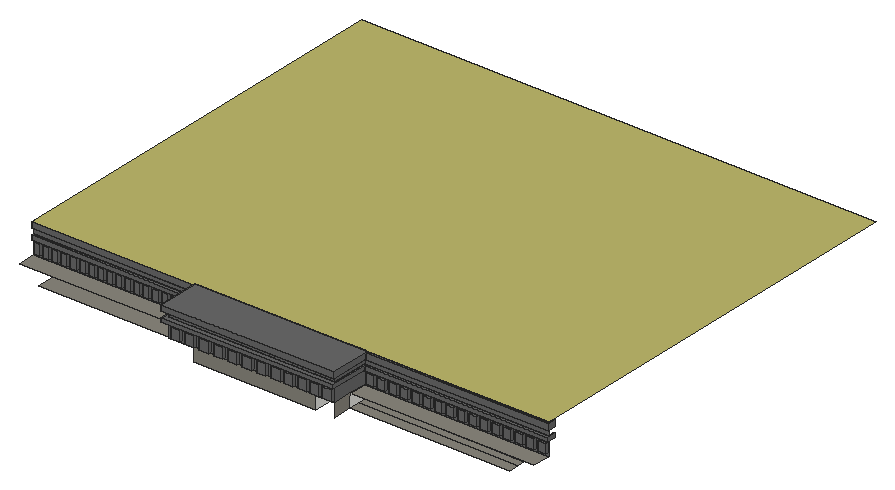
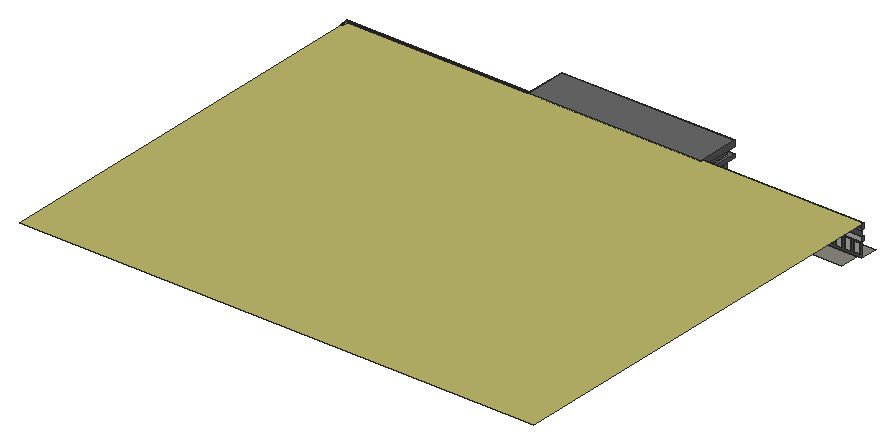
# SketchUp Ruby script. Lengths in inches.
U = 1.inch
M = Sketchup.active_model
def pt(a) = Geom::Point3d.new(a.map { |v| v * U })
def face(e, loops, mat)
  f = e.add_face(loops[0].map { |a| pt(a) })
  loops[1..].each { |l| e.add_face(l.map { |a| pt(a) }).erase! }
  f.material = f.back_material = mat if mat
  f
end
# faces: each face lists its corners as indices into pts; further lists are holes
def faces(e, pts, list, mat = nil) = list.each { |f| face(e, (f[0].is_a?(Array) ? f : [f]).map { |l| l.map { |i| pts[i] } }, mat) }
# xy, xz, yz: faces in a plane at the given z, y or x. An outline is a flat list of corners, or four numbers for a rectangle; further outlines are holes
def ring(l) = l.size == 4 ? [[l[0], l[1]], [l[2], l[1]], [l[2], l[3]], [l[0], l[3]]] : l.each_slice(2).to_a
def flat(e, list, mat, &to3) = list.each { |f| face(e, (f[0].is_a?(Array) ? f : [f]).map { |l| ring(l).map { |u, v| to3.(u, v) } }, mat) }
def xy(e, z, list, mat = nil) = flat(e, list, mat) { |x, y| [x, y, z] }
def xz(e, y, list, mat = nil) = flat(e, list, mat) { |x, z| [x, y, z] }
def yz(e, x, list, mat = nil) = flat(e, list, mat) { |y, z| [x, y, z] }
def lines(e, pts, list) = list.each { |a, b| e.add_line(pt(pts[a]), pt(pts[b])) }
# prism: a flat outline (further loops are holes) pulled along v
def prism(e, loops, v, mat = nil)
  f = face(e, loops, mat); d = Geom::Vector3d.new(v.map { |x| x * U })
  f.pushpull(f.normal.samedirection?(d) ? d.length : -d.length)
end
def box(e, o, s, mat = nil) = prism(e, [[o, [o[0] + s[0], o[1], o[2]], [o[0] + s[0], o[1] + s[1], o[2]], [o[0], o[1] + s[1], o[2]]]], [0, 0, s[2]], mat)
def at(x, y, z, deg = 0) = Geom::Transformation.translation(pt([x, y, z])) * Geom::Transformation.rotation(ORIGIN, Z_AXIS, deg.degrees)
def axes(o, x, y, z) = Geom::Transformation.new([*x, 0, *y, 0, *z, 0, *pt(o).to_a, 1])
def part(name) = M.definitions.add(name)
# library, detail: a bought-in or finely detailed component or shape, given as its bounding box
def library(name, o, s) = part(name).tap { |d| box(d.entities, o, s) }
def detail(e, o, s) = box(e.add_group.entities, o, s)
def put(e, d, t, mat = nil) = e.add_instance(d, t).tap { |i| i.material = mat if mat }
def group(e, t, mat = nil) = e.add_group.tap { |g| g.transformation = t; g.material = mat if mat }.entities
root = M.entities
M.materials.add("[0057_DarkKhaki]").color = [189, 183, 107]
M.materials.add("[0134_DimGray]").color = [105, 105, 105]
M.materials.add("[Formica Graystone]").color = [137, 134, 124]
xy(root,772.09,[[227.04,49.6875,370.55,104.375],[392.7,49.6875,580.01,80.4375]])
xy(root,772.09,[[227.04,6,370.55,49.6875],[27.68,28.6875,197.35,49.6875],[392.7,28.6875,580.01,40.6875],[392.7,40.6875,580.01,49.6875]],"[Formica Graystone]")
xy(root,787.6875,[[370.55,6,392.7,49.6875]])
xy(root,787.6875,[[4.9375,28.6875,197.35,49.6875],[392.7,28.6875,608.5,49.6875]],"[Formica Graystone]")
xy(root,789.48,[[202.16,3,213.03,6],[219.03,3,229.91,6],[235.91,3,246.78,6],[252.78,3,263.66,6],[269.66,3,280.53,6],
  [286.53,3,297.41,6],[303.41,3,314.28,6],[320.28,3,331.16,6],[335.41,3,346.28,6],[351.16,3,362.03,6],
  [365.72,3,376.6,6],[380.22,3,391.1,6]],"[0134_DimGray]")
xy(root,790.78,[[6.97,46.6875,14.16,49.6875],[17.66,46.6875,24.85,49.6875],[28.35,46.6875,35.54,49.6875],[39.04,46.6875,46.22,49.6875],[49.72,46.6875,56.91,49.6875],
  [60.41,46.6875,67.6,49.6875],[71.1,46.6875,78.29,49.6875],[81.79,46.6875,88.97,49.6875],[92.47,46.6875,99.66,49.6875],[103.16,46.6875,110.35,49.6875],
  [113.85,46.6875,121.04,49.6875],[124.54,46.6875,131.72,49.6875],[135.22,46.6875,142.41,49.6875],[145.91,46.6875,153.1,49.6875],[156.6,46.6875,163.79,49.6875],
  [167.29,46.6875,174.47,49.6875],[177.22,46.6875,184.41,49.6875],[187.66,46.6875,194.85,49.6875]])
xy(root,790.94,[[396.47,46.6875,405.6,49.6875],[409.91,46.6875,419.04,49.6875],[423.35,46.6875,432.47,49.6875],[436.79,46.6875,445.91,49.6875],[450.22,46.6875,459.35,49.6875],
  [463.66,46.6875,472.79,49.6875],[477.1,46.6875,486.22,49.6875],[490.54,46.6875,499.66,49.6875],[503.97,46.6875,513.1,49.6875],[517.41,46.6875,526.54,49.6875],
  [530.85,46.6875,539.97,49.6875],[544.29,46.6875,553.41,49.6875],[557.72,46.6875,566.85,49.6875],[571.16,46.6875,580.29,49.6875],[584.6,46.6875,593.72,49.6875],
  [598.04,46.6875,607.16,49.6875]])
xy(root,801.73,[[202.16,3,213.03,6],[219.03,3,229.91,6],[235.91,3,246.78,6],[252.78,3,263.66,6],[269.66,3,280.53,6],
  [286.53,3,297.41,6],[303.41,3,314.28,6],[320.28,3,331.16,6],[335.41,3,346.28,6],[351.16,3,362.03,6],
  [365.72,3,376.6,6],[380.22,3,391.1,6]],"[0134_DimGray]")
xy(root,802.13,[[396.47,46.6875,405.6,49.6875],[409.91,46.6875,419.04,49.6875],[423.35,46.6875,432.47,49.6875],[436.79,46.6875,445.91,49.6875],[450.22,46.6875,459.35,49.6875],
  [463.66,46.6875,472.79,49.6875],[477.1,46.6875,486.22,49.6875],[490.54,46.6875,499.66,49.6875],[503.97,46.6875,513.1,49.6875],[517.41,46.6875,526.54,49.6875],
  [530.85,46.6875,539.97,49.6875],[544.29,46.6875,553.41,49.6875],[557.72,46.6875,566.85,49.6875],[571.16,46.6875,580.29,49.6875],[584.6,46.6875,593.72,49.6875],
  [598.04,46.6875,607.16,49.6875]],"[0134_DimGray]")
xy(root,803.15,[[6.97,46.6875,14.16,49.6875],[17.66,46.6875,24.85,49.6875],[28.35,46.6875,35.54,49.6875],[39.04,46.6875,46.22,49.6875],[49.72,46.6875,56.91,49.6875],
  [60.41,46.6875,67.6,49.6875],[71.1,46.6875,78.29,49.6875],[81.79,46.6875,88.97,49.6875],[92.47,46.6875,99.66,49.6875],[103.16,46.6875,110.35,49.6875],
  [113.85,46.6875,121.04,49.6875],[124.54,46.6875,131.72,49.6875],[135.22,46.6875,142.41,49.6875],[145.91,46.6875,153.1,49.6875],[156.6,46.6875,163.79,49.6875],
  [167.29,46.6875,174.47,49.6875],[177.22,46.6875,184.41,49.6875],[187.66,46.6875,194.85,49.6875]],"[0134_DimGray]")
xy(root,804.58,[[395.2,46.6875,395.2,49.6875,608.5,49.6875,608.5,56.5625,610.0625,56.5625,610.0625,46.6875]],"[0134_DimGray]")
xy(root,804.73,[[4.9375,46.6875,193.85,49.6875]],"[0134_DimGray]")
xy(root,805.29,[[193.85,0,193.85,49.6875,197.35,49.6875,197.35,6,392.7,6,392.7,49.6875,395.2,49.6875,395.2,0]],"[0134_DimGray]")
xy(root,809.61,[[193.85,0,395.2,0,395.2,49.6875,392.7,49.6875,392.7,6,197.35,6,197.35,49.6875,193.85,49.6875],[4.9375,46.6875,193.85,49.6875],[395.2,46.6875,610.0625,46.6875,610.0625,56.5625,608.5,56.5625,608.5,49.6875,395.2,49.6875]],"[0134_DimGray]")
xy(root,816.49,[[396.39,46.6875,396.39,49.6875,608.5,49.6875,608.5,56.5625,610.75,56.5625,610.75,46.6875]],"[0134_DimGray]")
xy(root,816.9,[[193.79,0,193.79,49.6875,197.35,49.6875,197.35,6,392.7,6,392.7,49.6875,396.39,49.6875,396.39,0],[4.9375,46.6875,193.79,49.6875]],"[0134_DimGray]")
xy(root,823.6875,[[4.9375,46.6875,193.79,46.6875,193.79,49.6875,608.5,49.6875,608.5,529.6875,4.9375,529.6875]],"[0057_DarkKhaki]")
xy(root,823.6875,[[193.79,0,396.39,49.6875],[396.39,46.6875,610.75,46.6875,610.75,56.5625,608.5,56.5625,608.5,49.6875,396.39,49.6875]],"[0134_DimGray]")
xz(root,0,[[193.85,805.29,395.2,809.61],[193.79,816.9,396.39,823.6875]],"[0134_DimGray]")
xz(root,3,[[202.16,789.48,213.03,801.73],[219.03,789.48,229.91,801.73],[235.91,789.48,246.78,801.73],[252.78,789.48,263.66,801.73],[269.66,789.48,280.53,801.73],
  [286.53,789.48,297.41,801.73],[303.41,789.48,314.28,801.73],[320.28,789.48,331.16,801.73],[335.41,789.48,346.28,801.73],[351.16,789.48,362.03,801.73],
  [365.72,789.48,376.6,801.73],[380.22,789.48,391.1,801.73]],"[0134_DimGray]")
xz(root,6,[[197.35,805.29,392.7,809.61]])
xz(root,6,[[[197.35,787.6875,392.7,805.29],[202.16,789.48,213.03,801.73],[219.03,789.48,229.91,801.73],[235.91,789.48,246.78,801.73],[252.78,789.48,263.66,801.73],[269.66,789.48,280.53,801.73],[286.53,789.48,297.41,801.73],[303.41,789.48,314.28,801.73],[320.28,789.48,331.16,801.73],[335.41,789.48,346.28,801.73],[351.16,789.48,362.03,801.73],[365.72,789.48,376.6,801.73],[380.22,789.48,391.1,801.73]],[197.35,809.61,392.7,816.9]],"[0134_DimGray]")
xz(root,6,[[227.04,772.09,370.55,787.6875]],"[Formica Graystone]")
xz(root,46.6875,[[6.97,790.78,14.16,803.15],[17.66,790.78,24.85,803.15],[28.35,790.78,35.54,803.15],[39.04,790.78,46.22,803.15],[49.72,790.78,56.91,803.15],
  [60.41,790.78,67.6,803.15],[71.1,790.78,78.29,803.15],[81.79,790.78,88.97,803.15],[92.47,790.78,99.66,803.15],[103.16,790.78,110.35,803.15],
  [113.85,790.78,121.04,803.15],[124.54,790.78,131.72,803.15],[135.22,790.78,142.41,803.15],[145.91,790.78,153.1,803.15],[156.6,790.78,163.79,803.15],
  [167.29,790.78,174.47,803.15],[177.22,790.78,184.41,803.15],[187.66,790.78,194.85,803.15],[396.47,790.94,405.6,802.13],[409.91,790.94,419.04,802.13],
  [423.35,790.94,432.47,802.13],[436.79,790.94,445.91,802.13],[450.22,790.94,459.35,802.13],[463.66,790.94,472.79,802.13],[477.1,790.94,486.22,802.13],
  [490.54,790.94,499.66,802.13],[503.97,790.94,513.1,802.13],[517.41,790.94,526.54,802.13],[530.85,790.94,539.97,802.13],[544.29,790.94,553.41,802.13],
  [557.72,790.94,566.85,802.13],[571.16,790.94,580.29,802.13],[584.6,790.94,593.72,802.13],[598.04,790.94,607.16,802.13],[395.2,804.58,610.0625,809.61],
  [4.9375,804.73,193.85,809.61],[396.39,816.49,610.75,823.6875],[4.9375,816.9,193.79,823.6875]],"[0134_DimGray]")
xz(root,49.6875,[[197.35,772.09,224.47,787.6875],[224.47,772.09,226.6,787.6875],[226.6,772.09,227.04,787.6875],[370.55,772.09,370.74,787.6875],[370.74,772.09,374.55,787.6875],
  [374.55,772.09,392.7,787.6875],[197.35,787.6875,370.55,823.6875],[370.55,787.6875,370.74,823.6875],[370.74,787.6875,374.55,823.6875],[374.55,787.6875,392.7,823.6875],
  [6.97,790.78,14.16,803.15],[17.66,790.78,24.85,803.15],[28.35,790.78,35.54,803.15],[39.04,790.78,46.22,803.15],[49.72,790.78,56.91,803.15],
  [60.41,790.78,67.6,803.15],[71.1,790.78,78.29,803.15],[81.79,790.78,88.97,803.15],[92.47,790.78,99.66,803.15],[103.16,790.78,110.35,803.15],
  [113.85,790.78,121.04,803.15],[124.54,790.78,131.72,803.15],[135.22,790.78,142.41,803.15],[145.91,790.78,153.1,803.15],[156.6,790.78,163.79,803.15],
  [167.29,790.78,174.47,803.15],[177.22,790.78,184.41,803.15],[187.66,790.78,194.85,803.15],[409.91,790.94,419.04,802.13],[423.35,790.94,432.47,802.13],
  [436.79,790.94,445.91,802.13],[450.22,790.94,459.35,802.13],[463.66,790.94,472.79,802.13],[477.1,790.94,486.22,802.13],[490.54,790.94,499.66,802.13],
  [503.97,790.94,513.1,802.13],[517.41,790.94,526.54,802.13],[530.85,790.94,539.97,802.13],[544.29,790.94,553.41,802.13],[557.72,790.94,566.85,802.13],
  [571.16,790.94,580.29,802.13],[584.6,790.94,593.72,802.13],[598.04,790.94,607.16,802.13],[395.2,804.58,608.5,809.61],[4.9375,804.73,193.85,809.61],
  [193.85,805.29,197.35,809.61],[392.7,805.29,395.2,809.61],[396.39,816.49,608.5,823.6875],[193.79,816.9,197.35,823.6875],[392.7,816.9,396.39,823.6875]])
xz(root,49.6875,[[[4.9375,787.6875,197.35,787.6875,197.35,805.29,193.85,805.29,193.85,804.73,4.9375,804.73],[6.97,790.78,14.16,803.15],[17.66,790.78,24.85,803.15],[28.35,790.78,35.54,803.15],[39.04,790.78,46.22,803.15],[49.72,790.78,56.91,803.15],[60.41,790.78,67.6,803.15],[71.1,790.78,78.29,803.15],[81.79,790.78,88.97,803.15],[92.47,790.78,99.66,803.15],[103.16,790.78,110.35,803.15],[113.85,790.78,121.04,803.15],[124.54,790.78,131.72,803.15],[135.22,790.78,142.41,803.15],[145.91,790.78,153.1,803.15],[156.6,790.78,163.79,803.15],[167.29,790.78,174.47,803.15],[177.22,790.78,184.41,803.15],[187.66,790.78,194.85,803.15]],[[392.7,787.6875,608.5,787.6875,608.5,804.58,395.2,804.58,395.2,805.29,392.7,805.29],[396.47,790.94,405.6,802.13],[409.91,790.94,419.04,802.13],[423.35,790.94,432.47,802.13],[436.79,790.94,445.91,802.13],[450.22,790.94,459.35,802.13],[463.66,790.94,472.79,802.13],[477.1,790.94,486.22,802.13],[490.54,790.94,499.66,802.13],[503.97,790.94,513.1,802.13],[517.41,790.94,526.54,802.13],[530.85,790.94,539.97,802.13],[544.29,790.94,553.41,802.13],[557.72,790.94,566.85,802.13],[571.16,790.94,580.29,802.13],[584.6,790.94,593.72,802.13],[598.04,790.94,607.16,802.13]],[4.9375,809.61,197.35,816.9],[392.7,809.61,608.5,809.61,608.5,816.49,396.39,816.49,396.39,816.9,392.7,816.9]],"[0134_DimGray]")
xz(root,56.5625,[[608.5,804.58,610.0625,809.61],[608.5,816.49,610.75,823.6875]])
yz(root,4.9375,[[46.6875,804.73,49.6875,809.61],[46.6875,816.9,49.6875,823.6875]],"[0134_DimGray]")
yz(root,6.97,[[46.6875,790.78,49.6875,803.15]],"[0134_DimGray]")
yz(root,14.16,[[46.6875,790.78,49.6875,803.15]],"[0134_DimGray]")
yz(root,17.66,[[46.6875,790.78,49.6875,803.15]],"[0134_DimGray]")
yz(root,24.85,[[46.6875,790.78,49.6875,803.15]],"[0134_DimGray]")
yz(root,28.35,[[46.6875,790.78,49.6875,803.15]],"[0134_DimGray]")
yz(root,35.54,[[46.6875,790.78,49.6875,803.15]],"[0134_DimGray]")
yz(root,39.04,[[46.6875,790.78,49.6875,803.15]],"[0134_DimGray]")
yz(root,46.22,[[46.6875,790.78,49.6875,803.15]],"[0134_DimGray]")
yz(root,49.72,[[46.6875,790.78,49.6875,803.15]],"[0134_DimGray]")
yz(root,56.91,[[46.6875,790.78,49.6875,803.15]],"[0134_DimGray]")
yz(root,60.41,[[46.6875,790.78,49.6875,803.15]],"[0134_DimGray]")
yz(root,67.6,[[46.6875,790.78,49.6875,803.15]],"[0134_DimGray]")
yz(root,71.1,[[46.6875,790.78,49.6875,803.15]],"[0134_DimGray]")
yz(root,78.29,[[46.6875,790.78,49.6875,803.15]],"[0134_DimGray]")
yz(root,81.79,[[46.6875,790.78,49.6875,803.15]],"[0134_DimGray]")
yz(root,88.97,[[46.6875,790.78,49.6875,803.15]],"[0134_DimGray]")
yz(root,92.47,[[46.6875,790.78,49.6875,803.15]],"[0134_DimGray]")
yz(root,99.66,[[46.6875,790.78,49.6875,803.15]],"[0134_DimGray]")
yz(root,103.16,[[46.6875,790.78,49.6875,803.15]],"[0134_DimGray]")
yz(root,110.35,[[46.6875,790.78,49.6875,803.15]],"[0134_DimGray]")
yz(root,113.85,[[46.6875,790.78,49.6875,803.15]],"[0134_DimGray]")
yz(root,121.04,[[46.6875,790.78,49.6875,803.15]],"[0134_DimGray]")
yz(root,124.54,[[46.6875,790.78,49.6875,803.15]],"[0134_DimGray]")
yz(root,131.72,[[46.6875,790.78,49.6875,803.15]],"[0134_DimGray]")
yz(root,135.22,[[46.6875,790.78,49.6875,803.15]],"[0134_DimGray]")
yz(root,142.41,[[46.6875,790.78,49.6875,803.15]],"[0134_DimGray]")
yz(root,145.91,[[46.6875,790.78,49.6875,803.15]],"[0134_DimGray]")
yz(root,153.1,[[46.6875,790.78,49.6875,803.15]],"[0134_DimGray]")
yz(root,156.6,[[46.6875,790.78,49.6875,803.15]],"[0134_DimGray]")
yz(root,163.79,[[46.6875,790.78,49.6875,803.15]],"[0134_DimGray]")
yz(root,167.29,[[46.6875,790.78,49.6875,803.15]],"[0134_DimGray]")
yz(root,174.47,[[46.6875,790.78,49.6875,803.15]],"[0134_DimGray]")
yz(root,177.22,[[46.6875,790.78,49.6875,803.15]],"[0134_DimGray]")
yz(root,184.41,[[46.6875,790.78,49.6875,803.15]],"[0134_DimGray]")
yz(root,187.66,[[46.6875,790.78,49.6875,803.15]],"[0134_DimGray]")
yz(root,193.79,[[46.6875,816.9,49.6875,823.6875]])
yz(root,193.79,[[0,816.9,46.6875,823.6875]],"[0134_DimGray]")
yz(root,193.85,[[46.6875,804.73,49.6875,805.29],[46.6875,805.29,49.6875,809.61]])
yz(root,193.85,[[0,805.29,46.6875,809.61]],"[0134_DimGray]")
yz(root,194.85,[[46.6875,790.78,49.6875,803.15]])
yz(root,197.35,[[28.6875,772.09,49.6875,787.6875],[6,805.29,49.6875,809.61]])
yz(root,197.35,[[6,809.61,49.6875,816.9]],"[0134_DimGray]")
yz(root,202.16,[[3,789.48,6,801.73]],"[0134_DimGray]")
yz(root,213.03,[[3,789.48,6,801.73]],"[0134_DimGray]")
yz(root,219.03,[[3,789.48,6,801.73]],"[0134_DimGray]")
yz(root,229.91,[[3,789.48,6,801.73]],"[0134_DimGray]")
yz(root,235.91,[[3,789.48,6,801.73]],"[0134_DimGray]")
yz(root,246.78,[[3,789.48,6,801.73]],"[0134_DimGray]")
yz(root,252.78,[[3,789.48,6,801.73]],"[0134_DimGray]")
yz(root,263.66,[[3,789.48,6,801.73]],"[0134_DimGray]")
yz(root,269.66,[[3,789.48,6,801.73]],"[0134_DimGray]")
yz(root,280.53,[[3,789.48,6,801.73]],"[0134_DimGray]")
yz(root,286.53,[[3,789.48,6,801.73]],"[0134_DimGray]")
yz(root,297.41,[[3,789.48,6,801.73]],"[0134_DimGray]")
yz(root,303.41,[[3,789.48,6,801.73]],"[0134_DimGray]")
yz(root,314.28,[[3,789.48,6,801.73]],"[0134_DimGray]")
yz(root,320.28,[[3,789.48,6,801.73]],"[0134_DimGray]")
yz(root,331.16,[[3,789.48,6,801.73]],"[0134_DimGray]")
yz(root,335.41,[[3,789.48,6,801.73]],"[0134_DimGray]")
yz(root,346.28,[[3,789.48,6,801.73]],"[0134_DimGray]")
yz(root,351.16,[[3,789.48,6,801.73]],"[0134_DimGray]")
yz(root,362.03,[[3,789.48,6,801.73]],"[0134_DimGray]")
yz(root,365.72,[[3,789.48,6,801.73]],"[0134_DimGray]")
yz(root,370.55,[[6,772.09,49.6875,787.6875]])
yz(root,376.6,[[3,789.48,6,801.73]],"[0134_DimGray]")
yz(root,380.22,[[3,789.48,6,801.73]],"[0134_DimGray]")
yz(root,391.1,[[3,789.48,6,801.73]],"[0134_DimGray]")
yz(root,392.7,[[28.6875,772.09,49.6875,787.6875],[6,805.29,49.6875,809.61]])
yz(root,392.7,[[6,787.6875,49.6875,805.29],[6,809.61,49.6875,816.9]],"[0134_DimGray]")
yz(root,392.7,[[6,772.09,28.6875,787.6875]],"[Formica Graystone]")
yz(root,395.2,[[46.6875,804.58,49.6875,805.29],[46.6875,805.29,49.6875,809.61]])
yz(root,395.2,[[0,805.29,46.6875,809.61]],"[0134_DimGray]")
yz(root,396.39,[[46.6875,816.49,49.6875,816.9],[46.6875,816.9,49.6875,823.6875]])
yz(root,396.39,[[0,816.9,46.6875,823.6875]],"[0134_DimGray]")
yz(root,396.47,[[46.6875,790.94,49.6875,802.13]])
yz(root,405.6,[[46.6875,790.94,49.6875,802.13]],"[0134_DimGray]")
yz(root,409.91,[[46.6875,790.94,49.6875,802.13]],"[0134_DimGray]")
yz(root,419.04,[[46.6875,790.94,49.6875,802.13]],"[0134_DimGray]")
yz(root,423.35,[[46.6875,790.94,49.6875,802.13]],"[0134_DimGray]")
yz(root,432.47,[[46.6875,790.94,49.6875,802.13]],"[0134_DimGray]")
yz(root,436.79,[[46.6875,790.94,49.6875,802.13]],"[0134_DimGray]")
yz(root,445.91,[[46.6875,790.94,49.6875,802.13]],"[0134_DimGray]")
yz(root,450.22,[[46.6875,790.94,49.6875,802.13]],"[0134_DimGray]")
yz(root,459.35,[[46.6875,790.94,49.6875,802.13]],"[0134_DimGray]")
yz(root,463.66,[[46.6875,790.94,49.6875,802.13]],"[0134_DimGray]")
yz(root,472.79,[[46.6875,790.94,49.6875,802.13]],"[0134_DimGray]")
yz(root,477.1,[[46.6875,790.94,49.6875,802.13]],"[0134_DimGray]")
yz(root,486.22,[[46.6875,790.94,49.6875,802.13]],"[0134_DimGray]")
yz(root,490.54,[[46.6875,790.94,49.6875,802.13]],"[0134_DimGray]")
yz(root,499.66,[[46.6875,790.94,49.6875,802.13]],"[0134_DimGray]")
yz(root,503.97,[[46.6875,790.94,49.6875,802.13]],"[0134_DimGray]")
yz(root,513.1,[[46.6875,790.94,49.6875,802.13]],"[0134_DimGray]")
yz(root,517.41,[[46.6875,790.94,49.6875,802.13]],"[0134_DimGray]")
yz(root,526.54,[[46.6875,790.94,49.6875,802.13]],"[0134_DimGray]")
yz(root,530.85,[[46.6875,790.94,49.6875,802.13]],"[0134_DimGray]")
yz(root,539.97,[[46.6875,790.94,49.6875,802.13]],"[0134_DimGray]")
yz(root,544.29,[[46.6875,790.94,49.6875,802.13]],"[0134_DimGray]")
yz(root,553.41,[[46.6875,790.94,49.6875,802.13]],"[0134_DimGray]")
yz(root,557.72,[[46.6875,790.94,49.6875,802.13]],"[0134_DimGray]")
yz(root,566.85,[[46.6875,790.94,49.6875,802.13]],"[0134_DimGray]")
yz(root,571.16,[[46.6875,790.94,49.6875,802.13]],"[0134_DimGray]")
yz(root,580.29,[[46.6875,790.94,49.6875,802.13]],"[0134_DimGray]")
yz(root,584.6,[[46.6875,790.94,49.6875,802.13]],"[0134_DimGray]")
yz(root,593.72,[[46.6875,790.94,49.6875,802.13]],"[0134_DimGray]")
yz(root,598.04,[[46.6875,790.94,49.6875,802.13]],"[0134_DimGray]")
yz(root,607.16,[[46.6875,790.94,49.6875,802.13]],"[0134_DimGray]")
yz(root,608.5,[[49.6875,804.58,56.5625,809.61],[49.6875,816.49,56.5625,823.6875]])
yz(root,610.0625,[[46.6875,804.58,56.5625,809.61]],"[0134_DimGray]")
yz(root,610.75,[[46.6875,816.49,56.5625,823.6875]],"[0134_DimGray]")
p = [[392.7,6,816.9],[392.7,6,823.6875]]
lines(root,p,[[0,1]])
